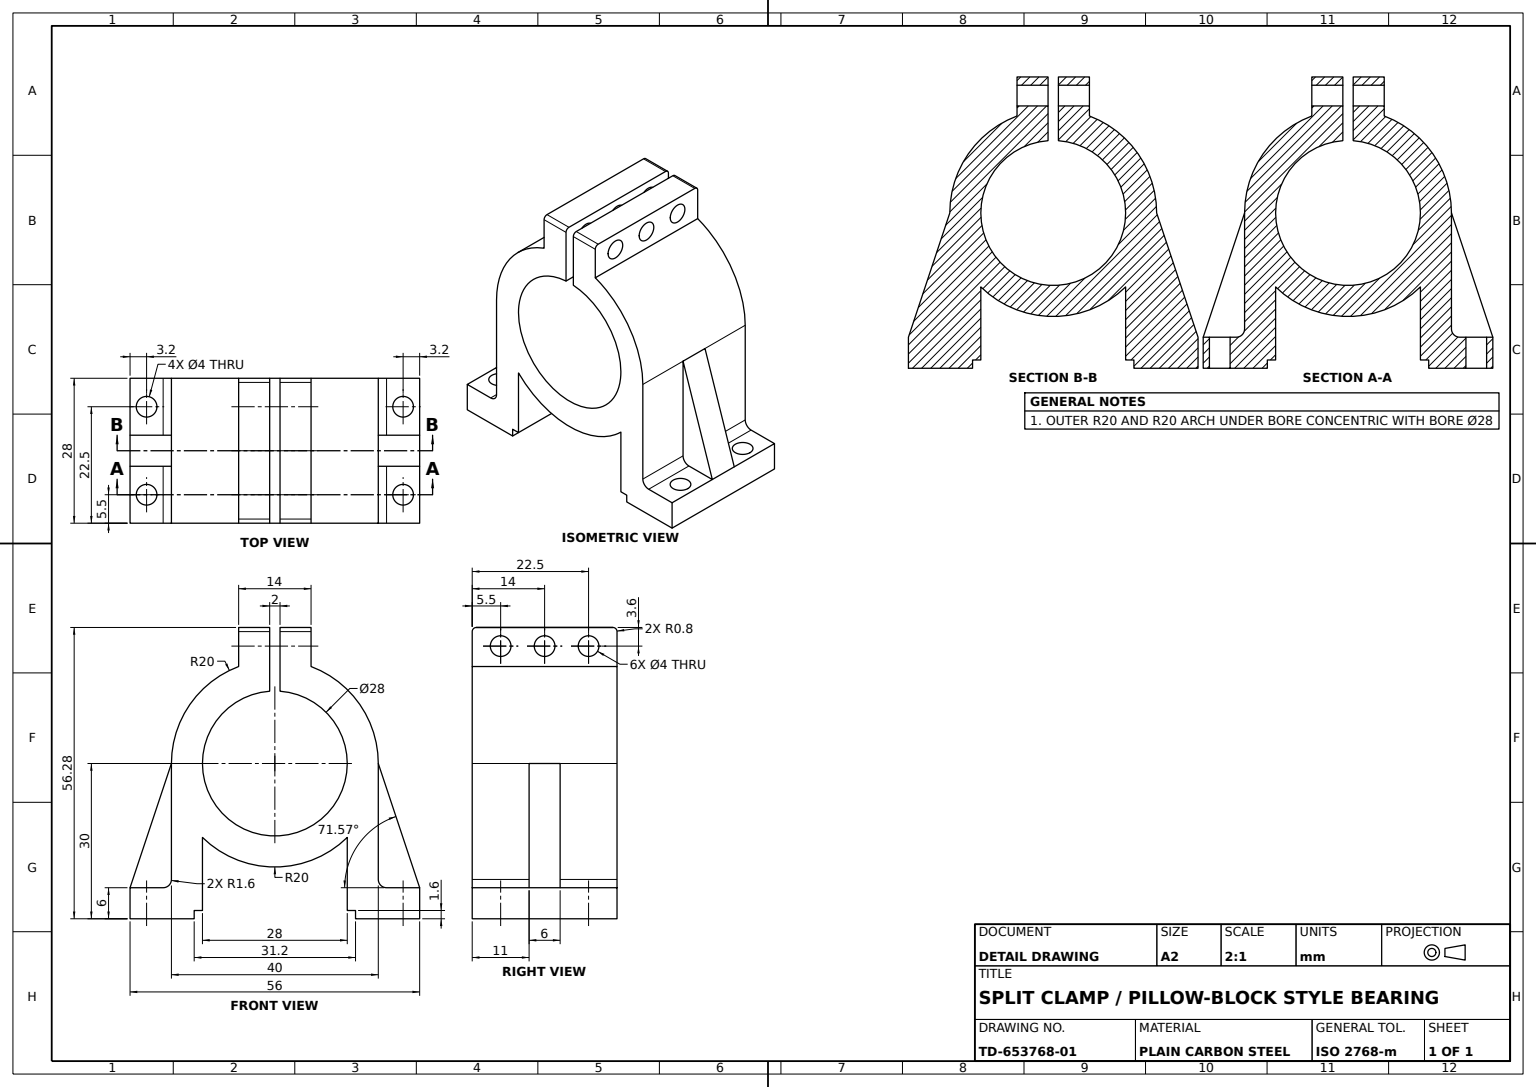
solid
v1 (-20,24,3)
v2 (-20,1.6,3)
e1 v1 v2 LINE
v3 (-20,1.6,14)
e2 v2 v3 LINE
v4 (-20,24,14)
e3 v4 v3 LINE
e4 v4 v1 LINE
face PLANE(AX(P(-20,0,14),D(1,0,0),D(0,1,0))) rev [e1 e2 -e3 e4]
v5 (1,50.278784,13.2)
v6 (7,50.278784,13.2)
e5 v5 v6 LINE
v7 (7,50.278784,-13.2)
e6 v7 v6 LINE
v8 (1,50.278784,-13.2)
e7 v7 v8 LINE
e8 v5 v8 LINE
face PLANE(AX(P(7,50.278784,-14),D(0,1,0),D(0,0,1))) [e5 -e6 e7 -e8]
v9 (-21.6,0,-3)
v10 (-28,0,-3)
e9 v9 v10 LINE
v11 (-20,24,-3)
e10 v11 v10 LINE
v12 (-20,1.6,-3)
e11 v11 v12 LINE
e12 v12 v9 CIRCLE(AX(P(-21.6,1.6,-3),D(0,0,-1),D(1,0,0)),1.6)
face PLANE(AX(P(0,22.139392,-3),D(0,0,1),D(1,0,0))) rev [e9 -e10 e11 e12]
v13 (-1,46.678784,-2)
v14 (-1,46.678784,2)
e13 v13 v14 CIRCLE(AX(P(-1,46.678784,0),D(-1,0,0),D(0,0,1)),2)
v15 (-7,46.678784,-2)
e14 v15 v13 LINE
v16 (-7,46.678784,2)
e15 v15 v16 CIRCLE(AX(P(-7,46.678784,0),D(-1,0,0),D(0,-1,0)),2)
e16 v16 v14 LINE
face CYL(AX(P(-45,46.678784,0),D(1,0,0),D(0,0,-1)),2) rev [-e13 -e14 e15 e16]
v17 (-1,50.278784,-13.2)
v18 (-7,50.278784,-13.2)
e17 v17 v18 LINE
v19 (-1,49.478784,-14)
e18 v19 v17 CIRCLE(AX(P(-1,49.478784,-13.2),D(1,0,0),D(0,0,1)),0.8)
v20 (-7,49.478784,-14)
e19 v20 v19 LINE
e20 v18 v20 CIRCLE(AX(P(-7,49.478784,-13.2),D(-1,0,0),D(0,-1,0)),0.8)
face CYL(AX(P(7,49.478784,-13.2),D(1,0,0),D(0,0,-1)),0.8) [-e17 -e18 -e19 -e20]
v21 (20,24,-3)
v22 (20,1.6,-3)
e21 v21 v22 LINE
v23 (20,1.6,-14)
e22 v22 v23 LINE
v24 (20,24,-14)
e23 v24 v23 LINE
e24 v21 v24 LINE
face PLANE(AX(P(20,0,14),D(1,0,0),D(0,1,0))) [e21 e22 -e23 -e24]
e25 v16 v15 CIRCLE(AX(P(-7,46.678784,0),D(-1,0,0),D(0,-1,0)),2)
v25 (-7,46.678784,6.5)
v26 (-7,46.678784,10.5)
e26 v25 v26 CIRCLE(AX(P(-7,46.678784,8.5),D(-1,0,0),D(0,-1,0)),2)
e27 v26 v25 CIRCLE(AX(P(-7,46.678784,8.5),D(-1,0,0),D(0,-1,0)),2)
v27 (-7,46.678784,-10.5)
v28 (-7,46.678784,-6.5)
e28 v27 v28 CIRCLE(AX(P(-7,46.678784,-8.5),D(-1,0,0),D(0,-1,0)),2)
e29 v28 v27 CIRCLE(AX(P(-7,46.678784,-8.5),D(-1,0,0),D(0,-1,0)),2)
v29 (-7,50.278784,13.2)
e30 v18 v29 LINE
v30 (-7,42.734994,-14)
e31 v20 v30 LINE
v31 (-7,42.734994,14)
e32 v31 v30 LINE
v32 (-7,49.478784,14)
e33 v32 v31 LINE
e34 v32 v29 CIRCLE(AX(P(-7,49.478784,13.2),D(-1,0,0),D(0,-1,0)),0.8)
face PLANE(AX(P(-7,50.278784,-14),D(-1,0,0),D(0,-1,0))) [-e25 -e15] [-e26 -e27] [-e28 -e29] [-e30 e20 e31 -e32 -e33 e34]
v33 (-1,46.678784,-6.5)
e35 v28 v33 LINE
v34 (-1,46.678784,-10.5)
e36 v34 v33 CIRCLE(AX(P(-1,46.678784,-8.5),D(-1,0,0),D(0,0,1)),2)
e37 v27 v34 LINE
face CYL(AX(P(-45,46.678784,-8.5),D(1,0,0),D(0,0,-1)),2) rev [e35 -e36 -e37 e28]
e38 v14 v13 CIRCLE(AX(P(-1,46.678784,0),D(-1,0,0),D(0,0,1)),2)
face CYL(AX(P(-45,46.678784,0),D(1,0,0),D(0,0,-1)),2) rev [-e38 -e16 e25 e14]
v35 (-26.8,-6,8.5)
v36 (-22.8,-6,8.5)
e39 v35 v36 CIRCLE(AX(P(-24.8,-6,8.5),D(0,1,0),D(0,0,1)),2)
v37 (-26.8,0,8.5)
e40 v35 v37 LINE
v38 (-22.8,0,8.5)
e41 v37 v38 CIRCLE(AX(P(-24.8,0,8.5),D(0,1,0),D(-1,0,0)),2)
e42 v36 v38 LINE
face CYL(AX(P(-24.8,-52,8.5),D(0,1,0),D(-1,0,0)),2) rev [-e39 e40 e41 -e42]
v39 (1,46.678784,-2)
v40 (1,46.678784,2)
e43 v39 v40 CIRCLE(AX(P(1,46.678784,0),D(1,0,0),D(0,0,-1)),2)
v41 (7,46.678784,-2)
e44 v39 v41 LINE
v42 (7,46.678784,2)
e45 v41 v42 CIRCLE(AX(P(7,46.678784,0),D(1,0,0),D(0,0,-1)),2)
e46 v40 v42 LINE
face CYL(AX(P(-45,46.678784,0),D(1,0,0),D(0,0,-1)),2) rev [-e43 e44 e45 -e46]
v43 (-21.6,0,-14)
v44 (-20,1.6,-14)
e47 v43 v44 CIRCLE(AX(P(-21.6,1.6,-14),D(0,0,1),D(1,0,0)),1.6)
e48 v9 v43 LINE
e49 v44 v12 LINE
face CYL(AX(P(-21.6,1.6,14),D(0,0,1),D(1,0,0)),1.6) rev [-e47 -e48 -e12 -e49]
v45 (14,24,14)
v46 (1,37.96424,14)
e50 v45 v46 CIRCLE(AX(P(0,24,14),D(0,0,1),D(1,0,0)),14)
v47 (1,37.96424,-14)
e51 v46 v47 LINE
v48 (14,24,-14)
e52 v48 v47 CIRCLE(AX(P(0,24,-14),D(0,0,1),D(1,0,0)),14)
e53 v48 v45 LINE
face CYL(AX(P(0,24,-82),D(0,0,1),D(1,0,0)),14) rev [e50 e51 -e52 e53]
v49 (22.8,-6,-8.5)
v50 (26.8,-6,-8.5)
e54 v49 v50 CIRCLE(AX(P(24.8,-6,-8.5),D(0,-1,0),D(1,0,0)),2)
e55 v50 v49 CIRCLE(AX(P(24.8,-6,-8.5),D(0,-1,0),D(1,0,0)),2)
v51 (22.8,-6,8.5)
v52 (26.8,-6,8.5)
e56 v51 v52 CIRCLE(AX(P(24.8,-6,8.5),D(0,-1,0),D(1,0,0)),2)
e57 v52 v51 CIRCLE(AX(P(24.8,-6,8.5),D(0,-1,0),D(1,0,0)),2)
v53 (28,-6,14)
v54 (28,-6,-14)
e58 v53 v54 LINE
v55 (15.6,-6,14)
e59 v53 v55 LINE
v56 (15.6,-6,-14)
e60 v55 v56 LINE
e61 v54 v56 LINE
face PLANE(AX(P(0,-6,14),D(0,-1,0),D(1,0,0))) [-e54 -e55] [-e56 -e57] [-e58 e59 e60 -e61]
e62 v42 v41 CIRCLE(AX(P(7,46.678784,0),D(1,0,0),D(0,0,-1)),2)
e63 v40 v39 CIRCLE(AX(P(1,46.678784,0),D(1,0,0),D(0,0,-1)),2)
face CYL(AX(P(-45,46.678784,0),D(1,0,0),D(0,0,-1)),2) rev [e62 -e44 -e63 e46]
v57 (22.8,0,-8.5)
v58 (26.8,0,-8.5)
e64 v57 v58 CIRCLE(AX(P(24.8,0,-8.5),D(0,1,0),D(-1,0,0)),2)
e65 v50 v58 LINE
e66 v49 v57 LINE
face CYL(AX(P(24.8,-52,-8.5),D(0,1,0),D(-1,0,0)),2) rev [e64 -e65 e55 e66]
v59 (-1,49.478784,14)
e67 v59 v32 LINE
v60 (-1,50.278784,13.2)
e68 v60 v59 CIRCLE(AX(P(-1,49.478784,13.2),D(1,0,0),D(0,0,1)),0.8)
e69 v29 v60 LINE
face CYL(AX(P(0,49.478784,13.2),D(-1,0,0),D(0,0,1)),0.8) [-e67 -e68 -e69 -e34]
v61 (28,0,-3)
e70 v61 v21 LINE
v62 (21.6,0,-3)
e71 v62 v61 LINE
e72 v62 v22 CIRCLE(AX(P(21.6,1.6,-3),D(0,0,-1),D(1,0,0)),1.6)
face PLANE(AX(P(0,22.139392,-3),D(0,0,1),D(1,0,0))) rev [-e70 -e71 e72 -e21]
e73 v38 v37 CIRCLE(AX(P(-24.8,0,8.5),D(0,1,0),D(-1,0,0)),2)
e74 v36 v35 CIRCLE(AX(P(-24.8,-6,8.5),D(0,1,0),D(0,0,1)),2)
face CYL(AX(P(-24.8,-52,8.5),D(0,1,0),D(-1,0,0)),2) rev [e42 e73 -e40 -e74]
v63 (1,46.678784,-6.5)
v64 (1,46.678784,-10.5)
e75 v63 v64 CIRCLE(AX(P(1,46.678784,-8.5),D(1,0,0),D(0,0,-1)),2)
v65 (7,46.678784,-6.5)
e76 v63 v65 LINE
v66 (7,46.678784,-10.5)
e77 v65 v66 CIRCLE(AX(P(7,46.678784,-8.5),D(1,0,0),D(0,0,-1)),2)
e78 v64 v66 LINE
face CYL(AX(P(-45,46.678784,-8.5),D(1,0,0),D(0,0,-1)),2) rev [-e75 e76 e77 -e78]
v67 (1,49.478784,-14)
e79 v47 v67 LINE
v68 (1,49.478784,14)
e80 v46 v68 LINE
e81 v68 v5 CIRCLE(AX(P(1,49.478784,13.2),D(-1,0,0),D(0,0,-1)),0.8)
e82 v8 v67 CIRCLE(AX(P(1,49.478784,-13.2),D(-1,0,0),D(0,0,-1)),0.8)
v69 (1,46.678784,10.5)
v70 (1,46.678784,6.5)
e83 v69 v70 CIRCLE(AX(P(1,46.678784,8.5),D(1,0,0),D(0,0,-1)),2)
e84 v70 v69 CIRCLE(AX(P(1,46.678784,8.5),D(1,0,0),D(0,0,-1)),2)
e85 v64 v63 CIRCLE(AX(P(1,46.678784,-8.5),D(1,0,0),D(0,0,-1)),2)
face PLANE(AX(P(1,38,-38),D(1,0,0),D(0,0,-1))) rev [e63 e43] [-e79 -e51 e80 e81 e8 e82] [e83 e84] [e75 e85]
v71 (-14,-4.4,14)
v72 (-14,-4.4,-14)
e86 v71 v72 LINE
v73 (-15.6,-4.4,14)
e87 v73 v71 LINE
v74 (-15.6,-4.4,-14)
e88 v73 v74 LINE
e89 v74 v72 LINE
face PLANE(AX(P(0,-4.4,14),D(0,1,0),D(0,0,1))) rev [-e86 -e87 e88 e89]
v75 (-14,24,14)
e90 v75 v45 CIRCLE(AX(P(0,24,14),D(0,0,1),D(1,0,0)),14)
v76 (-14,24,-14)
e91 v76 v48 CIRCLE(AX(P(0,24,-14),D(0,0,1),D(1,0,0)),14)
e92 v76 v75 LINE
face CYL(AX(P(0,24,-82),D(0,0,1),D(1,0,0)),14) rev [e90 -e53 -e91 e92]
v77 (28,0,14)
v78 (28,0,3)
e93 v77 v78 LINE
v79 (21.6,0,3)
e94 v79 v78 LINE
v80 (21.6,0,14)
e95 v79 v80 LINE
e96 v80 v77 LINE
v81 (22.8,0,8.5)
v82 (26.8,0,8.5)
e97 v81 v82 CIRCLE(AX(P(24.8,0,8.5),D(0,1,0),D(-1,0,0)),2)
e98 v82 v81 CIRCLE(AX(P(24.8,0,8.5),D(0,1,0),D(-1,0,0)),2)
face PLANE(AX(P(0,0,14),D(0,1,0),D(-1,0,0))) [e93 -e94 e95 e96] [-e97 -e98]
v83 (-15.6,-6,14)
e99 v83 v73 LINE
v84 (-15.6,-6,-14)
e100 v83 v84 LINE
e101 v84 v74 LINE
face PLANE(AX(P(-15.6,0,14),D(-1,0,0),D(0,0,1))) rev [-e88 -e99 e100 e101]
v85 (-1,37.96424,-14)
e102 v19 v85 LINE
e103 v17 v60 LINE
v86 (-1,37.96424,14)
e104 v59 v86 LINE
e105 v85 v86 LINE
v87 (-1,46.678784,6.5)
v88 (-1,46.678784,10.5)
e106 v87 v88 CIRCLE(AX(P(-1,46.678784,8.5),D(-1,0,0),D(0,0,1)),2)
e107 v88 v87 CIRCLE(AX(P(-1,46.678784,8.5),D(-1,0,0),D(0,0,1)),2)
e108 v33 v34 CIRCLE(AX(P(-1,46.678784,-8.5),D(-1,0,0),D(0,0,1)),2)
face PLANE(AX(P(-1,37.96424,-38),D(-1,0,0),D(0,0,1))) rev [e38 e13] [-e102 e18 e103 e68 e104 -e105] [e106 e107] [e36 e108]
v89 (-28,0,3)
e109 v1 v89 LINE
v90 (-21.6,0,3)
e110 v90 v89 LINE
e111 v2 v90 CIRCLE(AX(P(-21.6,1.6,3),D(0,0,-1),D(1,0,0)),1.6)
face PLANE(AX(P(0,22.139392,3),D(0,0,1),D(1,0,0))) [-e1 e109 -e110 -e111]
e112 v86 v75 CIRCLE(AX(P(0,24,14),D(0,0,1),D(1,0,0)),14)
e113 v85 v76 CIRCLE(AX(P(0,24,-14),D(0,0,1),D(1,0,0)),14)
face CYL(AX(P(0,24,-82),D(0,0,1),D(1,0,0)),14) rev [e112 -e92 -e113 e105]
v91 (7,49.478784,-14)
e114 v91 v7 CIRCLE(AX(P(7,49.478784,-13.2),D(1,0,0),D(0,0,-1)),0.8)
e115 v67 v91 LINE
face CYL(AX(P(7,49.478784,-13.2),D(1,0,0),D(0,0,-1)),0.8) [-e82 -e7 -e114 -e115]
e116 v78 v61 LINE
v92 (20,24,3)
e117 v92 v21 LINE
e118 v78 v92 LINE
face PLANE(AX(P(28,0,0),D(0.948683298,0.316227766,0),D(-0.316227766,0.948683298,0))) [e116 e70 -e117 -e118]
v93 (-21.6,0,14)
e119 v93 v90 LINE
e120 v3 v93 CIRCLE(AX(P(-21.6,1.6,14),D(0,0,-1),D(1,0,0)),1.6)
face CYL(AX(P(-21.6,1.6,14),D(0,0,1),D(1,0,0)),1.6) rev [e111 -e119 -e120 -e2]
v94 (-28,0,14)
e121 v94 v89 LINE
e122 v93 v94 LINE
face PLANE(AX(P(0,0,14),D(0,-1,0),D(1,0,0))) rev [-e73 -e41] [e119 e110 -e121 -e122]
v95 (7,46.678784,10.5)
e123 v69 v95 LINE
v96 (7,46.678784,6.5)
e124 v95 v96 CIRCLE(AX(P(7,46.678784,8.5),D(1,0,0),D(0,0,-1)),2)
e125 v70 v96 LINE
face CYL(AX(P(-45,46.678784,8.5),D(1,0,0),D(0,0,-1)),2) rev [-e83 e123 e124 -e125]
v97 (20,1.6,3)
e126 v79 v97 CIRCLE(AX(P(21.6,1.6,3),D(0,0,-1),D(1,0,0)),1.6)
v98 (20,1.6,14)
e127 v98 v97 LINE
e128 v80 v98 CIRCLE(AX(P(21.6,1.6,14),D(0,0,-1),D(1,0,0)),1.6)
face CYL(AX(P(21.6,1.6,14),D(0,0,1),D(1,0,0)),1.6) rev [-e95 e126 -e127 -e128]
v99 (20,24,14)
e129 v99 v92 LINE
e130 v99 v98 LINE
e131 v92 v97 LINE
face PLANE(AX(P(20,0,14),D(1,0,0),D(0,1,0))) [-e129 e130 e127 -e131]
v100 (-20,24,-14)
e132 v11 v100 LINE
e133 v100 v44 LINE
face PLANE(AX(P(-20,0,14),D(1,0,0),D(0,1,0))) rev [e132 e133 e49 -e11]
v101 (7,42.734994,14)
v102 (7,49.478784,14)
e134 v101 v102 LINE
e135 v102 v68 LINE
e136 v31 v4 CIRCLE(AX(P(0,24,14),D(0,0,1),D(1,0,0)),20)
v103 (-28,-6,14)
e137 v94 v103 LINE
e138 v103 v83 LINE
v104 (-14,9.717143,14)
e139 v71 v104 LINE
v105 (14,9.717143,14)
e140 v104 v105 CIRCLE(AX(P(0,24,14),D(0,0,1),D(1,0,0)),20)
v106 (14,-4.4,14)
e141 v106 v105 LINE
v107 (15.6,-4.4,14)
e142 v107 v106 LINE
e143 v55 v107 LINE
e144 v77 v53 LINE
e145 v99 v101 CIRCLE(AX(P(0,24,14),D(0,0,1),D(1,0,0)),20)
face PLANE(AX(P(0,0,14),D(0,0,1),D(1,0,0))) [e134 e135 -e80 -e50 -e90 -e112 -e104 e67 e33 e136 e3 e120 e122 e137 e138 e99 e87 e139 e140 -e141 -e142 -e143 -e59 -e144 -e96 e128 -e130 e145]
v108 (-28,0,-14)
e146 v43 v108 LINE
e147 v30 v100 CIRCLE(AX(P(0,24,-14),D(0,0,1),D(1,0,0)),20)
v109 (7,42.734994,-14)
e148 v109 v91 LINE
e149 v24 v109 CIRCLE(AX(P(0,24,-14),D(0,0,1),D(1,0,0)),20)
v110 (21.6,0,-14)
e150 v23 v110 CIRCLE(AX(P(21.6,1.6,-14),D(0,0,1),D(1,0,0)),1.6)
v111 (28,0,-14)
e151 v110 v111 LINE
e152 v111 v54 LINE
v112 (15.6,-4.4,-14)
e153 v56 v112 LINE
v113 (14,-4.4,-14)
e154 v112 v113 LINE
v114 (14,9.717143,-14)
e155 v113 v114 LINE
v115 (-14,9.717143,-14)
e156 v115 v114 CIRCLE(AX(P(0,24,-14),D(0,0,1),D(1,0,0)),20)
e157 v72 v115 LINE
v116 (-28,-6,-14)
e158 v116 v84 LINE
e159 v108 v116 LINE
face PLANE(AX(P(0,0,-14),D(0,0,1),D(1,0,0))) rev [-e146 e47 -e133 -e147 -e31 e19 e102 e113 e91 e52 e79 e115 -e148 -e149 e23 e150 e151 e152 e61 e153 e154 e155 -e156 -e157 -e89 -e101 -e158 -e159]
e160 v105 v114 LINE
e161 v106 v113 LINE
face PLANE(AX(P(14,0,14),D(-1,0,0),D(0,0,1))) [e141 e160 -e155 -e161]
e162 v89 v10 LINE
e163 v10 v108 LINE
e164 v103 v116 LINE
face PLANE(AX(P(-28,0,14),D(1,0,0),D(0,0,-1))) rev [-e137 e121 e162 e163 e159 -e164]
e165 v25 v87 LINE
e166 v26 v88 LINE
face CYL(AX(P(-45,46.678784,8.5),D(1,0,0),D(0,0,-1)),2) rev [-e106 -e165 e26 e166]
e167 v110 v62 LINE
face CYL(AX(P(21.6,1.6,14),D(0,0,1),D(1,0,0)),1.6) rev [-e22 -e72 -e167 -e150]
e168 v6 v102 CIRCLE(AX(P(7,49.478784,13.2),D(1,0,0),D(0,0,-1)),0.8)
face CYL(AX(P(0,49.478784,13.2),D(-1,0,0),D(0,0,1)),0.8) [-e81 -e135 -e168 -e5]
v117 (-22.8,-6,-8.5)
v118 (-22.8,0,-8.5)
e169 v117 v118 LINE
v119 (-26.8,-6,-8.5)
e170 v119 v117 CIRCLE(AX(P(-24.8,-6,-8.5),D(0,1,0),D(0,0,1)),2)
v120 (-26.8,0,-8.5)
e171 v119 v120 LINE
e172 v120 v118 CIRCLE(AX(P(-24.8,0,-8.5),D(0,1,0),D(-1,0,0)),2)
face CYL(AX(P(-24.8,-52,-8.5),D(0,1,0),D(-1,0,0)),2) rev [-e169 -e170 e171 e172]
e173 v104 v115 LINE
face CYL(AX(P(0,24,14),D(0,0,-1),D(-1,0,0)),20) [-e160 -e140 e173 e156]
e174 v117 v119 CIRCLE(AX(P(-24.8,-6,-8.5),D(0,1,0),D(0,0,1)),2)
e175 v118 v120 CIRCLE(AX(P(-24.8,0,-8.5),D(0,1,0),D(-1,0,0)),2)
face CYL(AX(P(-24.8,-52,-8.5),D(0,1,0),D(-1,0,0)),2) rev [-e174 e169 e175 -e171]
e176 v11 v1 LINE
face CYL(AX(P(0,24,14),D(0,0,-1),D(-1,0,0)),20) [e147 -e132 e176 -e4 -e136 e32]
e177 v58 v57 CIRCLE(AX(P(24.8,0,-8.5),D(0,1,0),D(-1,0,0)),2)
face CYL(AX(P(24.8,-52,-8.5),D(0,1,0),D(-1,0,0)),2) rev [e54 e65 e177 -e66]
face PLANE(AX(P(-20,24,0),D(-0.948683298,0.316227766,0),D(-0.316227766,-0.948683298,0))) [e10 -e162 -e109 -e176]
face PLANE(AX(P(7,50.278784,-14),D(0,1,0),D(0,0,1))) [-e103 e17 e30 e69]
face PLANE(AX(P(-14,0,14),D(-1,0,0),D(0,0,1))) rev [-e173 -e139 e86 e157]
e178 v61 v111 LINE
face PLANE(AX(P(0,0,14),D(0,1,0),D(-1,0,0))) [e167 e71 e178 -e151] [-e64 -e177]
e179 v107 v112 LINE
face PLANE(AX(P(0,-4.4,14),D(0,-1,0),D(0,0,-1))) [-e154 -e179 e142 e161]
e180 v109 v101 LINE
face CYL(AX(P(0,24,14),D(0,0,-1),D(-1,0,0)),20) [e24 e149 e180 -e145 e129 e117]
e181 v96 v95 CIRCLE(AX(P(7,46.678784,8.5),D(1,0,0),D(0,0,-1)),2)
face CYL(AX(P(-45,46.678784,8.5),D(1,0,0),D(0,0,-1)),2) rev [-e84 e125 e181 -e123]
face PLANE(AX(P(28,0,14),D(1,0,0),D(0,0,-1))) [-e93 e144 e58 -e152 -e178 -e116]
e182 v52 v82 LINE
e183 v51 v81 LINE
face CYL(AX(P(24.8,-52,8.5),D(0,1,0),D(-1,0,0)),2) rev [e182 e98 -e183 e56]
face CYL(AX(P(-45,46.678784,8.5),D(1,0,0),D(0,0,-1)),2) rev [-e166 e27 e165 -e107]
e184 v66 v65 CIRCLE(AX(P(7,46.678784,-8.5),D(1,0,0),D(0,0,-1)),2)
face CYL(AX(P(-45,46.678784,-8.5),D(1,0,0),D(0,0,-1)),2) rev [e184 -e76 -e85 e78]
face PLANE(AX(P(0,22.139392,3),D(0,0,1),D(1,0,0))) [e94 e118 e131 -e126]
face CYL(AX(P(24.8,-52,8.5),D(0,1,0),D(-1,0,0)),2) rev [e183 e97 -e182 e57]
face PLANE(AX(P(15.6,0,14),D(-1,0,0),D(0,0,1))) [-e153 -e60 e143 e179]
face CYL(AX(P(-45,46.678784,-8.5),D(1,0,0),D(0,0,-1)),2) rev [-e35 e29 e37 -e108]
face PLANE(AX(P(7,42.734994,-14),D(1,0,0),D(0,0,-1))) [-e62 -e45] [-e134 -e180 e148 e114 e6 e168] [-e181 -e124] [-e77 -e184]
face PLANE(AX(P(0,-6,14),D(0,1,0),D(0,0,1))) rev [e174 e170] [-e100 -e138 e164 e158] [e39 e74]
face PLANE(AX(P(0,0,14),D(0,-1,0),D(1,0,0))) rev [-e175 -e172] [-e9 e48 e146 -e163]
